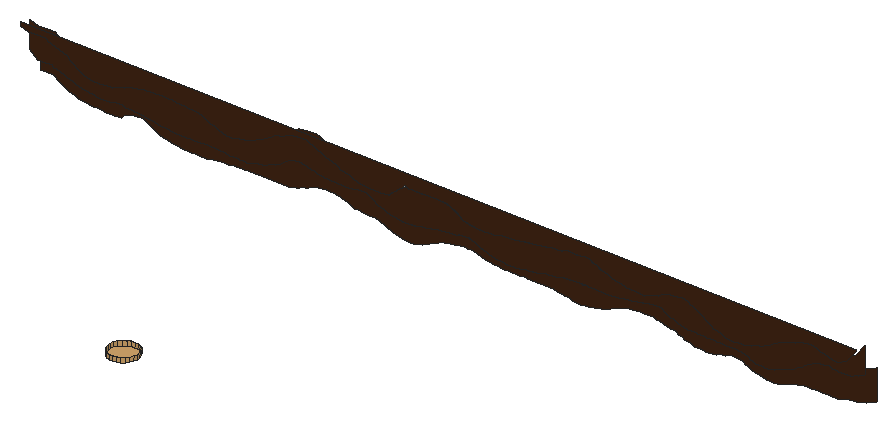
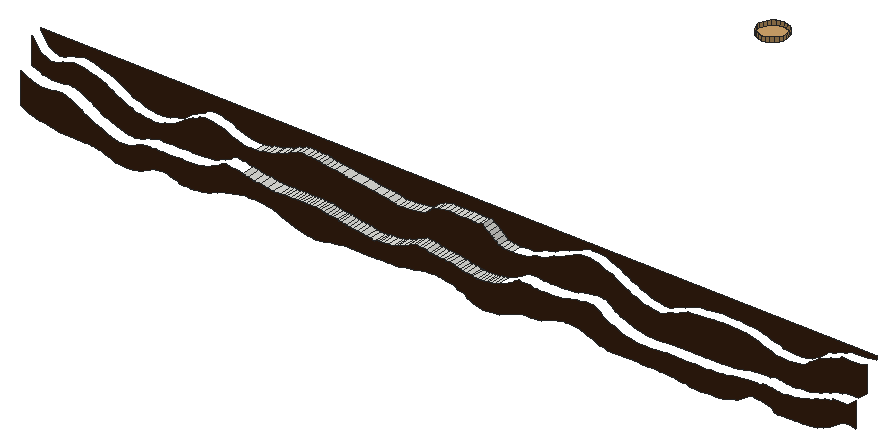
# SketchUp Ruby script. Lengths in inches.
U = 1.inch
M = Sketchup.active_model
def pt(a) = Geom::Point3d.new(a.map { |v| v * U })
def face(e, loops, mat)
  f = e.add_face(loops[0].map { |a| pt(a) })
  loops[1..].each { |l| e.add_face(l.map { |a| pt(a) }).erase! }
  f.material = f.back_material = mat if mat
  f
end
# faces: each face lists its corners as indices into pts; further lists are holes
def faces(e, pts, list, mat = nil) = list.each { |f| face(e, (f[0].is_a?(Array) ? f : [f]).map { |l| l.map { |i| pts[i] } }, mat) }
# xy, xz, yz: faces in a plane at the given z, y or x. An outline is a flat list of corners, or four numbers for a rectangle; further outlines are holes
def ring(l) = l.size == 4 ? [[l[0], l[1]], [l[2], l[1]], [l[2], l[3]], [l[0], l[3]]] : l.each_slice(2).to_a
def flat(e, list, mat, &to3) = list.each { |f| face(e, (f[0].is_a?(Array) ? f : [f]).map { |l| ring(l).map { |u, v| to3.(u, v) } }, mat) }
def xy(e, z, list, mat = nil) = flat(e, list, mat) { |x, y| [x, y, z] }
def xz(e, y, list, mat = nil) = flat(e, list, mat) { |x, z| [x, y, z] }
def yz(e, x, list, mat = nil) = flat(e, list, mat) { |y, z| [x, y, z] }
def lines(e, pts, list) = list.each { |a, b| e.add_line(pt(pts[a]), pt(pts[b])) }
# prism: a flat outline (further loops are holes) pulled along v
def prism(e, loops, v, mat = nil)
  f = face(e, loops, mat); d = Geom::Vector3d.new(v.map { |x| x * U })
  f.pushpull(f.normal.samedirection?(d) ? d.length : -d.length)
end
def box(e, o, s, mat = nil) = prism(e, [[o, [o[0] + s[0], o[1], o[2]], [o[0] + s[0], o[1] + s[1], o[2]], [o[0], o[1] + s[1], o[2]]]], [0, 0, s[2]], mat)
def at(x, y, z, deg = 0) = Geom::Transformation.translation(pt([x, y, z])) * Geom::Transformation.rotation(ORIGIN, Z_AXIS, deg.degrees)
def axes(o, x, y, z) = Geom::Transformation.new([*x, 0, *y, 0, *z, 0, *pt(o).to_a, 1])
def part(name) = M.definitions.add(name)
# library, detail: a bought-in or finely detailed component or shape, given as its bounding box
def library(name, o, s) = part(name).tap { |d| box(d.entities, o, s) }
def detail(e, o, s) = box(e.add_group.entities, o, s)
def put(e, d, t, mat = nil) = e.add_instance(d, t).tap { |i| i.material = mat if mat }
def group(e, t, mat = nil) = e.add_group.tap { |g| g.transformation = t; g.material = mat if mat }.entities
root = M.entities
M.materials.add("[Field Square Tile]").color = [211, 167, 108]
M.materials.add("[Wood Veneer 01]").color = [66, 38, 20]
xy(root,243.05,[[358.29,563.18,358.97,565.74]])
xy(root,243.07,[[356.4375,563.18,357.02,565.74]])
xy(root,243.09,[[353.125,563.18,353.65,565.74],[353.65,563.18,354.17,565.74],[354.17,563.18,354.83,565.74],[354.83,563.18,355.28,565.74]])
xy(root,249.21,[[325.92,561.05,326.81,563.18]])
xy(root,249.22,[[327.53,561.05,328.4375,563.18]])
xy(root,249.23,[[329.08,561.05,329.98,563.18]])
xy(root,250.6875,[[324.47,492.77,323.81,492.86,323.19,493.11,322.66,493.52,322.25,494.05,322,494.67,321.91,495.33,322,495.99,322.25,496.61,322.66,497.14,323.19,497.55,323.81,497.81,324.47,497.89,325.13,497.81,325.75,497.55,326.28,497.14,326.69,496.61,326.95,495.99,327.03,495.33,326.95,494.67,326.69,494.05,326.28,493.52,325.75,493.11,325.13,492.86]],"[Field Square Tile]")
xz(root,561.05,[[384.34,244.87,385.25,245.01,386.1875,245.12,386.95,245.25,387.71,245.41,388.34,245.78,389.14,245.88,389.85,246.16,390.45,246.57,391.24,246.9,391.84,247.35,392.51,247.62,393.1,248.06,393.86,248.32,394.97,248.66,395.75,248.79,396.61,249.19,397.28,249.32,398.21,249.41,399.06,249.48,399.81,249.21,400.45,248.96,401.15,248.9,401.95,248.42,402.66,248.3,403.37,248.22,404.1875,248.56,405.12,249.02,406.85,251.16,406.85,251.5,252.84,251.5,252.84,250.88,254.43,250.53,256.05,250.54,257.51,250.55,258.04,250.15,258.65,249.97,259.45,249.8,260.12,249.41,260.79,249.2,261.56,249.01,262.05,248.51,262.68,248.07,263.33,247.72,263.97,247.25,264.52,246.88,265.24,246.73,265.9,246.62,266.64,246.54,267.42,246.51,268.2,246.58,269,246.59,269.8,246.69,270.51,247.03,271.2,247.2,272.17,247.39,272.8,247.78,273.58,247.89,274.58,248.18,275.22,248.29,276.11,248.35,276.84,248.4,277.83,248.4375,278.49,248.46,279.38,248.47,280.12,248.48,281.01,248.49,281.74,248.39,283.14,248.28,284.17,248.15,284.99,248.11,285.79,248.08,286.63,247.66,287.26,247.46,287.94,247.08,288.625,246.94,289.48,246.66,290.09,246.35,290.86,246.05,291.76,246.13,292.47,246.29,293.27,246.41,294.18,246.55,294.91,246.92,295.52,247.12,296.2,247.31,296.77,247.71,297.7,248.03,298.41,248.46,299.19,248.82,299.91,249.37,300.7,249.5625,301.6,249.9,302.52,250.35,303.18,250.49,303.99,250.6,305.01,250.58,305.65,250.61,306.27,250.32,306.96,250.0625,307.62,249.68,308.38,249.46,309.27,248.95,310.49,248.69,311.4,248.26,312,247.9,313.13,247.66,313.71,247.53,314.39,247.25,315.2,246.95,315.89,246.75,316.68,246.66,317.39,246.59,318.28,246.55,319.21,246.63,319.95,246.74,320.68,246.87,321.29,247.42,321.96,247.96,322.53,248.44,323.27,248.85,323.74,249.34,324.47,249.125,325.24,249.17,325.92,249.21,326.81,249.21,327.53,249.22,328.4375,249.22,329.08,249.23,329.98,249.23,330.72,249.24,331.52,249.14,332.15,248.82,332.94,248.54,333.64,248.04,334.33,247.48,335.22,247.29,336.04,247.15,336.77,247.05,337.49,247,338.4,246.96,339.125,246.94,340.04,247.04,341.1,247.36,342.28,247.43,343.93,247.6,345.91,247.98,348.11,248.1875,349.72,248.49,350.97,248.62,351.91,248.69,352.59,248.75,353.25,249.09,353.95,249.18,354.73,249.13,355.43,249.17,356.13,249.18,357.03,249.29,357.76,249.21,358.37,248.8,359.0625,248.73,359.84,248.26,360.54,248.02,361.34,247.8125,362.05,247.4,362.96,247.27,363.7,247.18,364.625,246.91,365.49,246.84,366.44,246.79,367.22,246.75,367.97,246.83,369.01,247.25,369.88,247.55,370.55,247.66,371.18,248.16,371.97,248.41,372.67,248.52,373.37,248.72,374.07,248.8,374.96,248.85,375.79,248.6875,376.33,248.26,377.02,248.06,377.91,247.55,378.62,247.19,379.43,246.63,380.0625,246.13,380.65,245.83,381.33,245.67,382.2,245.46,382.91,245.0625,383.625,244.95]],"[Wood Veneer 01]")
xz(root,563.18,[[388.34,241.09,388.91,241.14,389.55,241.35,390.14,241.46,391.08,241.85,392.08,242.23,392.64,242.42,393.36,242.61,393.875,242.91,394.25,243.14,394.79,243.52,395.27,243.71,395.6,244.02,396.04,244.21,396.63,244.57,397.1,244.76,397.72,245.125,398.22,245.32,398.7,245.41,399.25,245.48,399.74,245.59,400.27,245.55,400.88,245.35,401.37,245.31,401.92,245.27,402.48,245.24,403.04,245.22,403.6,245.34,404.23,245.42,404.8125,245.52,405.19,245.76,405.66,245.9,406.85,246.43,406.85,251.16,405.12,249.02,404.1875,248.56,403.37,248.22,402.66,248.3,401.95,248.42,401.15,248.9,400.45,248.96,399.81,249.21,399.06,249.48,398.21,249.41,397.28,249.32,396.61,249.19,395.75,248.79,394.97,248.66,393.86,248.32,393.1,248.06,392.51,247.62,391.84,247.35,391.24,246.9,390.45,246.57,389.85,246.16,389.14,245.88,388.34,245.78,387.71,245.41,386.95,245.25,386.1875,245.12,385.25,245.01,384.34,244.87,383.625,244.95,382.91,245.0625,382.2,245.46,381.33,245.67,380.65,245.83,380.0625,246.13,379.43,246.63,378.62,247.19,377.91,247.55,377.02,248.06,376.33,248.26,375.79,248.6875,374.96,248.85,374.07,248.8,373.37,248.72,372.67,248.52,371.97,248.41,371.18,248.16,370.55,247.66,369.88,247.55,369.01,247.25,367.97,246.83,367.22,246.75,366.44,246.79,365.49,246.84,364.625,246.91,363.7,247.18,362.96,247.27,362.05,247.4,361.34,247.8125,360.54,248.02,359.84,248.26,359.0625,248.73,358.37,248.8,357.76,249.21,357.03,249.29,356.13,249.18,355.43,249.17,354.73,249.13,353.95,249.18,353.25,249.09,352.59,248.75,351.91,248.69,350.97,248.62,349.72,248.49,348.11,248.1875,345.91,247.98,343.93,247.6,342.28,247.43,341.1,247.36,340.04,247.04,339.125,246.94,338.4,246.96,337.49,247,336.77,247.05,336.04,247.15,335.22,247.29,334.33,247.48,333.64,248.04,332.94,248.54,332.15,248.82,331.52,249.14,330.72,249.24,329.98,249.23,329.08,249.23,328.4375,249.22,327.53,249.22,326.81,249.21,325.92,249.21,325.24,249.17,324.47,249.125,323.74,249.34,323.27,248.85,322.53,248.44,321.96,247.96,321.29,247.42,320.68,246.87,319.95,246.74,319.21,246.63,318.28,246.55,317.39,246.59,316.68,246.66,315.89,246.75,315.2,246.95,314.39,247.25,313.71,247.53,313.13,247.66,312,247.9,311.4,248.26,310.49,248.69,309.27,248.95,308.38,249.46,307.62,249.68,306.96,250.0625,306.27,250.32,305.65,250.61,305.01,250.58,303.99,250.6,303.18,250.49,302.52,250.35,301.6,249.9,300.7,249.5625,299.91,249.37,299.19,248.82,298.41,248.46,297.7,248.03,296.77,247.71,296.2,247.31,295.52,247.12,294.91,246.92,294.18,246.55,293.27,246.41,292.47,246.29,291.76,246.13,290.86,246.05,290.09,246.35,289.48,246.66,288.625,246.94,287.94,247.08,287.26,247.46,286.63,247.66,285.79,248.08,284.99,248.11,284.17,248.15,283.14,248.28,281.74,248.39,281.01,248.49,280.12,248.48,279.38,248.47,278.49,248.46,277.83,248.4375,276.84,248.4,276.11,248.35,275.22,248.29,274.58,248.18,273.58,247.89,272.8,247.78,272.17,247.39,271.2,247.2,270.51,247.03,269.8,246.69,269,246.59,268.2,246.58,267.42,246.51,266.64,246.54,265.9,246.62,265.24,246.73,264.52,246.88,263.97,247.25,263.33,247.72,262.68,248.07,262.05,248.51,261.56,249.01,260.79,249.2,260.12,249.41,259.45,249.8,258.65,249.97,258.04,250.15,257.51,250.55,256.05,250.54,254.43,250.53,252.84,250.88,252.84,246.2,254.41,244.96,255.8,244.9375,257.05,244.92,257.27,244.61,257.83,244.54,258.59,244.41,259.26,244.11,259.78,243.95,260.44,243.79,260.96,243.48,261.6,243.3,262.1875,243.14,262.67,243.06,263.39,242.85,263.97,242.78,264.78,242.73,265.32,242.68,265.99,242.51,266.51,242.46,267.05,242.58,267.68,242.57,268.31,242.81,268.88,242.86,269.44,242.89,270.08,242.92,270.51,242.625,271.12,242.65,271.67,242.62,272.3,242.58,272.86,242.57,273.5,242.48,274.16,242.38,274.82,242.34,275.49,242.24,276.66,241.96,277.43,241.89,278.25,241.83,278.85,241.78,279.62,241.75,280.07,241.74,280.62,241.72,281.88,241.7,282.61,241.69,283.28,241.68,283.87,241.68,284.36,241.67,285.0625,241.74,285.63,241.75,287.63,241.75,288.12,241.67,288.65,241.66,289.26,241.57,289.8,241.53,290.42,241.51,290.97,241.49,291.67,241.48,292.33,241.47,292.9,241.46,293.61,241.6,294.34,241.85,295.01,241.91,295.91,242.1,296.68,242.46,297.38,242.78,298.15,242.97,298.68,243.23,299.08,243.48,299.6,243.72,299.9375,244.12,300.41,244.39,300.89,244.73,301.375,244.87,301.96,244.95,302.64,245.01,303.29,244.81,303.86,244.7,304.34,244.67,304.95,244.55,305.49,244.51,305.95,244.25,306.7,244.11,307.26,244.04,307.88,243.99,308.6,243.95,309.1,243.93,309.79,243.91,310.36,243.89,311.06,243.88,311.71,243.94,312.35,243.95,312.91,244.1,313.54,244.13,314.02,244.15,314.54,244.17,315.06,244.18,315.66,243.8,316.2,243.43,316.81,243.09,317.2,242.875,317.7,242.68,318.29,242.51,318.8,242.21,319.4,242.11,320.08,241.96,320.64,241.89,321.1,241.85,321.62,241.8125,322.13,241.79,322.71,241.78,323.38,241.91,323.85,241.93,324.52,242.09,325.29,242.2,325.79,242.24,326.4,242.42,326.95,242.47,327.7,242.71,328.34,242.78,328.82,242.82,329.51,242.85,330.21,242.87,330.76,243.02,331.38,243.05,331.93,243.29,332.61,243.35,333.16,243.39,333.76,243.42,334.53,243.14,335.1,242.9375,335.65,242.65,336.27,242.39,337.03,242.14,337.67,241.89,338.16,241.78,339.21,241.63,339.98,241.56,340.58,241.51,341.03,241.48,341.55,241.46,342.42,241.51,343.14,241.59,344.08,241.82,344.86,241.87,345.625,241.98,346.24,242.02,346.89,242.19,347.59,242.38,348.08,242.4375,348.6,242.48,349.26,242.58,349.79,242.61,350.375,242.77,350.83,242.95,351.39,243.01,351.9,243.05,352.47,243.08,353.125,243.09,355.28,243.09,355.85,243.08,356.4375,243.07,357.02,243.07,357.68,243.0625,358.29,243.05,358.97,243.05,360.24,243.1,361.41,243.17,362.55,243.4,363.8125,243.52,364.94,243.71,365.84,243.99,366.54,244.08,367.24,244.21,367.82,244.27,368.36,244.3,369.03,244.39,369.625,244.19,370,243.88,370.48,243.59,371.03,243.33,371.58,243.22,372.07,242.92,372.55,242.75,373.11,242.6,373.67,242.52,374.23,242.47,374.8125,242.43,375.39,242.4,375.97,242.39,376.55,242.37,377.13,242.36,377.72,242.35,378.88,242.33,379.46,242.33,380.18,242.32,380.65,242.3125,381.29,242.3,381.96,242.3,382.41,242.29,383.05,242.28,383.5625,242.28,384.19,242.2,384.77,241.97,385.34,241.84,385.85,241.57,386.27,241.33,386.74,241.24,387.27,241.17,387.74,241.12]],"[Wood Veneer 01]")
xz(root,565.74,[[321.7,236.98,322.38,237.22,323.23,237.43,323.85,237.74,324.55,238.02,324.99,238.375,325.55,238.51,326.1875,238.76,326.83,239.12,327.41,239.22,328.41,239.31,329.22,239.54,329.71,239.6,330.33,239.65,330.92,239.69,331.48,239.7,332.21,239.72,332.82,239.56,333.49,239.44,334.34,239.16,334.89,239.07,335.66,238.93,336.54,238.78,337.02,238.73,337.69,238.6875,338.38,238.66,339.05,238.65,339.83,238.64,340.45,238.63,341.14,238.625,342,238.625,342.56,238.62,347.45,238.62,348.14,238.45,348.9,238.25,349.52,238.19,350.29,238.15,350.92,237.86,351.69,237.79,352.4,237.74,353.27,237.87,353.92,237.88,355.04,238.14,356.26,238.46,357.01,238.72,357.89,239.08,358.68,239.375,359.42,239.75,360.07,239.97,360.69,240.17,361.37,240.27,362.05,240.33,362.74,240.37,363.43,240.4,364.125,240.41,364.65,240.42,365.23,240.43,365.8,240.43,366.45,240.27,367.03,240.23,367.68,239.96,368.4375,239.8,369.05,239.65,369.8125,239.5,370.4375,239.18,371.12,239.01,371.64,238.67,372.21,238.56,372.87,238.48,373.4375,238.26,374.01,238.19,374.83,238.15,375.36,238.11,376.03,238.18,376.71,238.18,377.39,238.27,377.91,238.55,378.57,238.61,379.16,238.66,379.73,239.04,380.47,239.125,381.15,239.02,381.84,238.96,382.36,238.86,382.86,238.57,383.41,238.33,384.12,238,384.95,237.71,385.49,237.59,386.09,237.51,386.68,237.45,387.25,237.42,387.98,237.4,388.66,237.47,389.26,237.5625,389.95,237.84,390.63,238.08,391.32,238.33,391.85,238.51,392.42,238.6,393.08,238.74,393.66,238.8,394.23,238.83,394.97,238.86,395.73,238.875,396.27,238.88,396.95,238.89,397.63,238.89,398.39,238.9,399.78,238.9,400.41,239.15,401.18,239.28,401.98,239.42,402.7,239.49,403.25,239.53,403.9375,239.81,404.46,239.96,405.02,240.1,406.85,240.89,406.85,246.43,405.66,245.9,405.19,245.76,404.8125,245.52,404.23,245.42,403.6,245.34,403.04,245.22,402.48,245.24,401.92,245.27,401.37,245.31,400.88,245.35,400.27,245.55,399.74,245.59,399.25,245.48,398.7,245.41,398.22,245.32,397.72,245.125,397.1,244.76,396.63,244.57,396.04,244.21,395.6,244.02,395.27,243.71,394.79,243.52,394.25,243.14,393.875,242.91,393.36,242.61,392.64,242.42,392.08,242.23,391.08,241.85,390.14,241.46,389.55,241.35,388.91,241.14,388.34,241.09,387.74,241.12,387.27,241.17,386.74,241.24,386.27,241.33,385.85,241.57,385.34,241.84,384.77,241.97,384.19,242.2,383.5625,242.28,383.05,242.28,382.41,242.29,381.96,242.3,381.29,242.3,380.65,242.3125,380.18,242.32,379.46,242.33,378.88,242.33,377.72,242.35,377.13,242.36,376.55,242.37,375.97,242.39,375.39,242.4,374.8125,242.43,374.23,242.47,373.67,242.52,373.11,242.6,372.55,242.75,372.07,242.92,371.58,243.22,371.03,243.33,370.48,243.59,370,243.88,369.625,244.19,369.03,244.39,368.36,244.3,367.82,244.27,367.24,244.21,366.54,244.08,365.84,243.99,364.94,243.71,363.8125,243.52,362.55,243.4,361.41,243.17,360.24,243.1,358.97,243.05,358.29,243.05,357.68,243.0625,357.02,243.07,356.4375,243.07,355.85,243.08,355.28,243.09,353.125,243.09,352.47,243.08,351.9,243.05,351.39,243.01,350.83,242.95,350.375,242.77,349.79,242.61,349.26,242.58,348.6,242.48,348.08,242.4375,347.59,242.38,346.89,242.19,346.24,242.02,345.625,241.98,344.86,241.87,344.08,241.82,343.14,241.59,342.42,241.51,341.55,241.46,341.03,241.48,340.58,241.51,339.98,241.56,339.21,241.63,338.16,241.78,337.67,241.89,337.03,242.14,336.27,242.39,335.65,242.65,335.1,242.9375,334.53,243.14,333.76,243.42,333.16,243.39,332.61,243.35,331.93,243.29,331.38,243.05,330.76,243.02,330.21,242.87,329.51,242.85,328.82,242.82,328.34,242.78,327.7,242.71,326.95,242.47,326.4,242.42,325.79,242.24,325.29,242.2,324.52,242.09,323.85,241.93,323.38,241.91,322.71,241.78,322.13,241.79,321.62,241.8125,321.1,241.85,320.64,241.89,320.08,241.96,319.4,242.11,318.8,242.21,318.29,242.51,317.7,242.68,317.2,242.875,316.81,243.09,316.2,243.43,315.66,243.8,315.06,244.18,314.54,244.17,314.02,244.15,313.54,244.13,312.91,244.1,312.35,243.95,311.71,243.94,311.06,243.88,310.36,243.89,309.79,243.91,309.1,243.93,308.6,243.95,307.88,243.99,307.26,244.04,306.7,244.11,305.95,244.25,305.49,244.51,304.95,244.55,304.34,244.67,303.86,244.7,303.29,244.81,302.64,245.01,301.96,244.95,301.375,244.87,300.89,244.73,300.41,244.39,299.9375,244.12,299.6,243.72,299.08,243.48,298.68,243.23,298.15,242.97,297.38,242.78,296.68,242.46,295.91,242.1,295.01,241.91,294.34,241.85,293.61,241.6,292.9,241.46,292.33,241.47,291.67,241.48,290.97,241.49,290.42,241.51,289.8,241.53,289.26,241.57,288.65,241.66,288.12,241.67,287.63,241.75,285.63,241.75,285.0625,241.74,284.36,241.67,283.87,241.68,283.28,241.68,282.61,241.69,281.88,241.7,280.62,241.72,280.07,241.74,279.62,241.75,278.85,241.78,278.25,241.83,277.43,241.89,276.66,241.96,275.49,242.24,274.82,242.34,274.16,242.38,273.5,242.48,272.86,242.57,272.3,242.58,271.67,242.62,271.12,242.65,270.51,242.625,270.08,242.92,269.44,242.89,268.88,242.86,268.31,242.81,267.68,242.57,267.05,242.58,266.51,242.46,265.99,242.51,265.32,242.68,264.78,242.73,263.97,242.78,263.39,242.85,262.67,243.06,262.1875,243.14,261.6,243.3,260.96,243.48,260.44,243.79,259.78,243.95,259.26,244.11,258.59,244.41,257.83,244.54,257.27,244.61,257.05,244.92,255.8,244.9375,254.41,244.96,252.84,246.2,252.84,241.52,254.05,241.69,255.32,241.55,256.34,240.85,256.88,240.59,257.48,240.2,258.27,239.86,258.72,239.64,259.28,239.52,259.79,239.19,260.57,239.09,261.26,239.03,261.94,238.97,262.64,238.94,263.34,238.93,264.03,238.92,265.07,238.82,265.58,238.8,266.45,238.79,267.19,238.77,267.72,238.9375,268.28,239.55,268.86,239.69,269.41,239.88,270.14,239.99,270.73,240.05,271.39,240.09,272.08,240.11,272.78,239.71,273.24,239.38,273.82,239.11,274.4,238.74,275.05,238.43,275.96,238.31,276.43,238.21,277.37,237.9,278.03,237.82,278.72,237.76,279.43,237.71,280.04,237.68,280.64,237.67,281.39,237.66,282.08,237.65,283.39,237.65,284.06,237.89,284.82,237.94,285.4375,237.98,286.29,238.1,286.84,238.13,287.6,238.15,288.23,238.26,288.98,238.28,289.61,238.3,290.46,238.32,291.18,238.33,292.41,238.33,293.09,238.34,298.66,238.34,299.17,238.59,299.99,238.72,300.68,238.86,301.19,239.18,301.78,239.35,302.34,239.52,302.89,239.85,303.53,240.03,304.1875,240.12,304.86,240.19,305.625,240.23,306.33,240.25,306.95,240.27,307.73,240.11,308.36,239.92,309.05,239.7,309.58,239.53,310.16,239.29,310.82,239.04,311.4,238.94,311.97,238.875,312.72,238.83,313.48,238.8,314.02,238.79,314.69,238.78,315.47,238.43,316.25,238.28,316.8125,237.96,317.75,237.68,318.42,237.33,318.95,237.2,319.64,237.11,320.4,237.04,321.09,237.01]],"[Wood Veneer 01]")
p = [[339.98,563.18,241.56],[339.98,565.74,241.56],[340.58,565.74,241.51],[340.58,563.18,241.51],[341.03,565.74,241.48],[341.03,563.18,241.48],
  [341.55,565.74,241.46],[341.55,563.18,241.46],[342.42,565.74,241.51],[342.42,563.18,241.51],[343.14,565.74,241.59],[343.14,563.18,241.59],
  [338.16,563.18,241.78],[338.16,565.74,241.78],[339.21,565.74,241.63],[339.21,563.18,241.63],[344.08,565.74,241.82],[344.08,563.18,241.82],
  [320.64,563.18,241.89],[320.64,565.74,241.89],[321.1,565.74,241.85],[321.1,563.18,241.85],[321.62,565.74,241.8125],[321.62,563.18,241.8125],
  [322.13,565.74,241.79],[322.13,563.18,241.79],[322.71,565.74,241.78],[322.71,563.18,241.78],[323.38,565.74,241.91],[323.38,563.18,241.91],
  [337.67,563.18,241.89],[337.67,565.74,241.89],[344.86,565.74,241.87],[344.86,563.18,241.87],[320.08,563.18,241.96],[320.08,565.74,241.96],
  [323.85,565.74,241.93],[323.85,563.18,241.93],[324.52,565.74,242.09],[324.52,563.18,242.09],[337.03,563.18,242.14],[337.03,565.74,242.14],
  [345.625,565.74,241.98],[345.625,563.18,241.98],[319.4,563.18,242.11],[319.4,565.74,242.11],[346.24,565.74,242.02],[346.24,563.18,242.02],
  [346.89,565.74,242.19],[346.89,563.18,242.19],[318.8,563.18,242.21],[318.8,565.74,242.21],[325.29,565.74,242.2],[325.29,563.18,242.2],
  [336.27,563.18,242.39],[336.27,565.74,242.39],[325.79,565.74,242.24],[325.79,563.18,242.24],[326.4,565.74,242.42],[326.4,563.18,242.42],
  [347.59,565.74,242.38],[347.59,563.18,242.38],[326.95,565.74,242.47],[326.95,563.18,242.47],[335.65,563.18,242.65],[335.65,565.74,242.65],
  [348.08,565.74,242.4375],[348.08,563.18,242.4375],[348.6,565.74,242.48],[348.6,563.18,242.48],[327.7,565.74,242.71],[327.7,563.18,242.71],
  [349.26,565.74,242.58],[349.26,563.18,242.58],[335.1,563.18,242.9375],[335.1,565.74,242.9375],[349.79,565.74,242.61],[349.79,563.18,242.61],
  [350.375,565.74,242.77],[350.375,563.18,242.77],[328.34,565.74,242.78],[328.34,563.18,242.78],[328.82,565.74,242.82],[328.82,563.18,242.82],
  [329.51,565.74,242.85],[329.51,563.18,242.85],[350.83,565.74,242.95],[350.83,563.18,242.95],[330.21,565.74,242.87],[330.21,563.18,242.87],
  [330.76,565.74,243.02],[330.76,563.18,243.02],[334.53,563.18,243.14],[334.53,565.74,243.14],[331.38,565.74,243.05],[331.38,563.18,243.05],
  [351.39,565.74,243.01],[351.39,563.18,243.01],[351.9,565.74,243.05],[351.9,563.18,243.05],[352.47,565.74,243.08],[352.47,563.18,243.08],
  [358.97,563.18,243.05],[358.97,565.74,243.05],[360.24,565.74,243.1],[360.24,563.18,243.1],[331.93,565.74,243.29],[331.93,563.18,243.29],
  [333.76,563.18,243.42],[333.76,565.74,243.42],[353.125,565.74,243.09],[353.125,563.18,243.09],[355.28,563.18,243.09],[355.28,565.74,243.09],
  [355.85,565.74,243.08],[355.85,563.18,243.08],[356.4375,565.74,243.07],[356.4375,563.18,243.07],[357.02,563.18,243.07],[357.02,565.74,243.07],
  [357.68,565.74,243.0625],[357.68,563.18,243.0625],[358.29,565.74,243.05],[358.29,563.18,243.05],[361.41,565.74,243.17],[361.41,563.18,243.17],
  [362.55,565.74,243.4],[362.55,563.18,243.4],[332.61,565.74,243.35],[332.61,563.18,243.35],[333.16,565.74,243.39],[333.16,563.18,243.39],
  [363.8125,565.74,243.52],[363.8125,563.18,243.52],[364.94,565.74,243.71],[364.94,563.18,243.71],[365.84,565.74,243.99],[365.84,563.18,243.99],
  [318.28,561.05,246.55],[318.28,563.18,246.55],[319.21,563.18,246.63],[319.21,561.05,246.63],[319.95,563.18,246.74],[319.95,561.05,246.74],
  [320.68,563.18,246.87],[320.68,561.05,246.87],[364.625,561.05,246.91],[364.625,563.18,246.91],[365.49,563.18,246.84],[365.49,561.05,246.84],
  [321.29,563.18,247.42],[321.29,561.05,247.42],[338.4,561.05,246.96],[338.4,563.18,246.96],[339.125,563.18,246.94],[339.125,561.05,246.94],
  [340.04,563.18,247.04],[340.04,561.05,247.04],[363.7,561.05,247.18],[363.7,563.18,247.18],[336.04,561.05,247.15],[336.04,563.18,247.15],
  [336.77,563.18,247.05],[336.77,561.05,247.05],[337.49,563.18,247],[337.49,561.05,247],[341.1,563.18,247.36],[341.1,561.05,247.36],
  [335.22,561.05,247.29],[335.22,563.18,247.29],[362.96,561.05,247.27],[362.96,563.18,247.27],[334.33,561.05,247.48],[334.33,563.18,247.48],
  [362.05,561.05,247.4],[362.05,563.18,247.4],[321.96,563.18,247.96],[321.96,561.05,247.96],[342.28,563.18,247.43],[342.28,561.05,247.43],
  [343.93,563.18,247.6],[343.93,561.05,247.6],[361.34,561.05,247.8125],[361.34,563.18,247.8125],[333.64,561.05,248.04],[333.64,563.18,248.04],
  [345.91,563.18,247.98],[345.91,561.05,247.98],[360.54,561.05,248.02],[360.54,563.18,248.02],[322.53,563.18,248.44],[322.53,561.05,248.44],
  [332.94,561.05,248.54],[332.94,563.18,248.54],[348.11,563.18,248.1875],[348.11,561.05,248.1875],[359.84,561.05,248.26],[359.84,563.18,248.26],
  [349.72,563.18,248.49],[349.72,561.05,248.49],[359.0625,561.05,248.73],[359.0625,563.18,248.73],[323.27,563.18,248.85],[323.27,561.05,248.85],
  [332.15,561.05,248.82],[332.15,563.18,248.82],[350.97,563.18,248.62],[350.97,561.05,248.62],[351.91,563.18,248.69],[351.91,561.05,248.69],
  [352.59,563.18,248.75],[352.59,561.05,248.75],[358.37,561.05,248.8],[358.37,563.18,248.8],[331.52,561.05,249.14],[331.52,563.18,249.14],
  [353.25,563.18,249.09],[353.25,561.05,249.09],[357.76,561.05,249.21],[357.76,563.18,249.21],[323.74,563.18,249.34],[323.74,561.05,249.34],
  [324.47,563.18,249.125],[324.47,561.05,249.125],[325.24,563.18,249.17],[325.24,561.05,249.17],[330.72,561.05,249.24],[330.72,563.18,249.24],
  [353.95,563.18,249.18],[353.95,561.05,249.18],[354.73,563.18,249.13],[354.73,561.05,249.13],[355.43,563.18,249.17],[355.43,561.05,249.17],
  [325.92,563.18,249.21],[325.92,561.05,249.21],[326.81,561.05,249.21],[326.81,563.18,249.21],[327.53,563.18,249.22],[327.53,561.05,249.22],
  [328.4375,561.05,249.22],[328.4375,563.18,249.22],[329.08,563.18,249.23],[329.08,561.05,249.23],[329.98,561.05,249.23],[329.98,563.18,249.23],
  [356.13,563.18,249.18],[356.13,561.05,249.18],[357.03,563.18,249.29],[357.03,561.05,249.29],[324.47,492.77,251.5],[323.81,492.86,251.5],
  [323.81,492.86,250.6875],[324.47,492.77,250.6875],[325.13,492.86,251.5],[325.13,492.86,250.6875],[323.19,493.11,251.5],[323.19,493.11,250.6875],
  [325.75,493.11,251.5],[325.75,493.11,250.6875],[322.66,493.52,251.5],[322.66,493.52,250.6875],[326.28,493.52,251.5],[326.28,493.52,250.6875],
  [322.25,494.05,251.5],[322.25,494.05,250.6875],[326.69,494.05,251.5],[326.69,494.05,250.6875],[322,494.67,251.5],[322,494.67,250.6875],
  [326.95,494.67,251.5],[326.95,494.67,250.6875],[321.91,495.33,251.5],[321.91,495.33,250.6875],[327.03,495.33,251.5],[327.03,495.33,250.6875],
  [322,495.99,251.5],[322,495.99,250.6875],[326.95,495.99,251.5],[326.95,495.99,250.6875],[322.25,496.61,251.5],[322.25,496.61,250.6875],
  [326.69,496.61,251.5],[326.69,496.61,250.6875],[322.66,497.14,251.5],[322.66,497.14,250.6875],[326.28,497.14,251.5],[326.28,497.14,250.6875],
  [323.19,497.55,251.5],[323.19,497.55,250.6875],[325.75,497.55,251.5],[325.75,497.55,250.6875],[323.81,497.81,251.5],[323.81,497.81,250.6875],
  [325.13,497.81,251.5],[325.13,497.81,250.6875],[324.47,497.89,251.5],[324.47,497.89,250.6875]]
faces(root,p,[[0,1,2,3],[3,2,4,5],[5,4,6,7],[7,6,8,9],[9,8,10,11],[12,13,14,15],[15,14,1,0],[11,10,16,17],
  [18,19,20,21],[21,20,22,23],[23,22,24,25],[25,24,26,27],[27,26,28,29],[30,31,13,12],[17,16,32,33],[34,35,19,18],
  [29,28,36,37],[37,36,38,39],[40,41,31,30],[33,32,42,43],[44,45,35,34],[43,42,46,47],[47,46,48,49],[50,51,45,44],
  [39,38,52,53],[54,55,41,40],[53,52,56,57],[57,56,58,59],[49,48,60,61],[59,58,62,63],[64,65,55,54],[61,60,66,67],
  [67,66,68,69],[63,62,70,71],[69,68,72,73],[74,75,65,64],[73,72,76,77],[77,76,78,79],[71,70,80,81],[81,80,82,83],
  [83,82,84,85],[79,78,86,87],[85,84,88,89],[89,88,90,91],[92,93,75,74],[91,90,94,95],[87,86,96,97],[97,96,98,99],
  [99,98,100,101],[102,103,104,105],[95,94,106,107],[108,109,93,92],[101,100,110,111],[112,113,114,115],[115,114,116,117],[118,119,120,121],
  [121,120,122,123],[105,104,124,125],[125,124,126,127],[107,106,128,129],[129,128,130,131],[131,130,109,108],[127,126,132,133],[133,132,134,135],
  [135,134,136,137],[138,139,140,141],[141,140,142,143],[143,142,144,145],[146,147,148,149],[145,144,150,151],[152,153,154,155],[155,154,156,157],
  [158,159,147,146],[160,161,162,163],[163,162,164,165],[165,164,153,152],[157,156,166,167],[168,169,161,160],[170,171,159,158],[172,173,169,168],
  [174,175,171,170],[151,150,176,177],[167,166,178,179],[179,178,180,181],[182,183,175,174],[184,185,173,172],[181,180,186,187],[188,189,183,182],
  [177,176,190,191],[192,193,185,184],[187,186,194,195],[196,197,189,188],[195,194,198,199],[200,201,197,196],[191,190,202,203],[204,205,193,192],
  [199,198,206,207],[207,206,208,209],[209,208,210,211],[212,213,201,200],[214,215,205,204],[211,210,216,217],[218,219,213,212],[203,202,220,221],
  [221,220,222,223],[223,222,224,225],[226,227,215,214],[217,216,228,229],[229,228,230,231],[231,230,232,233],[225,224,234,235],[236,237,238,239],
  [240,241,242,243],[244,245,227,226],[233,232,246,247],[247,246,248,249],[249,248,219,218]])
faces(root,p,[[250,251,252,253],[254,250,253,255],[251,256,257,252],[258,254,255,259],[256,260,261,257],[262,258,259,263],[260,264,265,261],[266,262,263,267],
  [264,268,269,265],[270,266,267,271],[268,272,273,269],[274,270,271,275],[272,276,277,273],[278,274,275,279],[276,280,281,277],[282,278,279,283],
  [280,284,285,281],[286,282,283,287],[284,288,289,285],[290,286,287,291],[288,292,293,289],[294,290,291,295],[292,296,297,293],[296,294,295,297]],"[Field Square Tile]")
